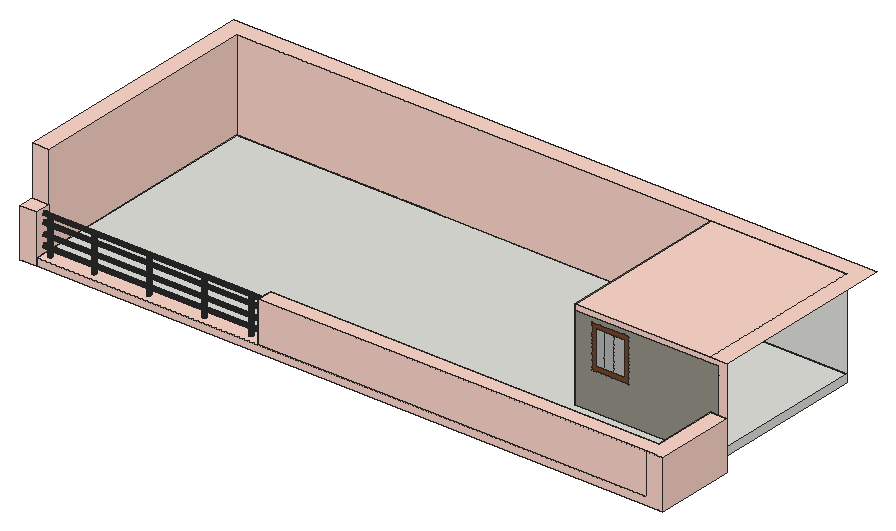
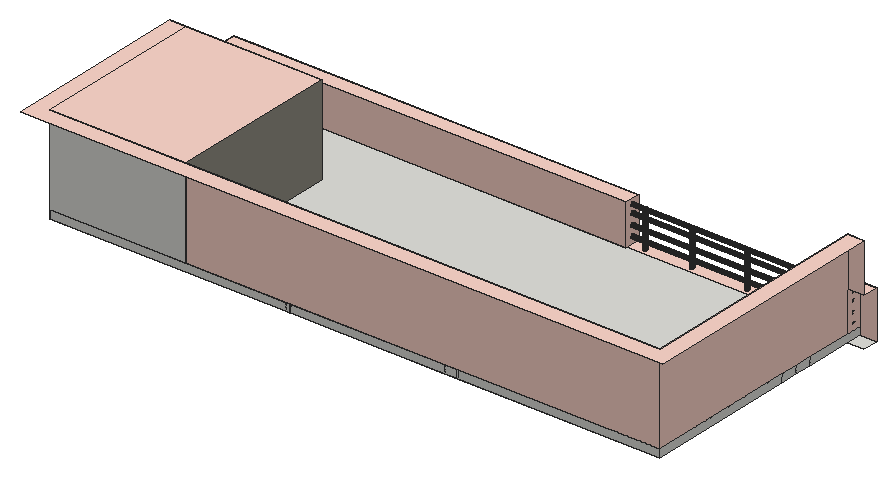
# SketchUp Ruby script. Lengths in inches.
U = 1.inch
M = Sketchup.active_model
def pt(a) = Geom::Point3d.new(a.map { |v| v * U })
def face(e, loops, mat)
  f = e.add_face(loops[0].map { |a| pt(a) })
  loops[1..].each { |l| e.add_face(l.map { |a| pt(a) }).erase! }
  f.material = f.back_material = mat if mat
  f
end
# faces: each face lists its corners as indices into pts; further lists are holes
def faces(e, pts, list, mat = nil) = list.each { |f| face(e, (f[0].is_a?(Array) ? f : [f]).map { |l| l.map { |i| pts[i] } }, mat) }
# xy, xz, yz: faces in a plane at the given z, y or x. An outline is a flat list of corners, or four numbers for a rectangle; further outlines are holes
def ring(l) = l.size == 4 ? [[l[0], l[1]], [l[2], l[1]], [l[2], l[3]], [l[0], l[3]]] : l.each_slice(2).to_a
def flat(e, list, mat, &to3) = list.each { |f| face(e, (f[0].is_a?(Array) ? f : [f]).map { |l| ring(l).map { |u, v| to3.(u, v) } }, mat) }
def xy(e, z, list, mat = nil) = flat(e, list, mat) { |x, y| [x, y, z] }
def xz(e, y, list, mat = nil) = flat(e, list, mat) { |x, z| [x, y, z] }
def yz(e, x, list, mat = nil) = flat(e, list, mat) { |y, z| [x, y, z] }
def lines(e, pts, list) = list.each { |a, b| e.add_line(pt(pts[a]), pt(pts[b])) }
# prism: a flat outline (further loops are holes) pulled along v
def prism(e, loops, v, mat = nil)
  f = face(e, loops, mat); d = Geom::Vector3d.new(v.map { |x| x * U })
  f.pushpull(f.normal.samedirection?(d) ? d.length : -d.length)
end
def box(e, o, s, mat = nil) = prism(e, [[o, [o[0] + s[0], o[1], o[2]], [o[0] + s[0], o[1] + s[1], o[2]], [o[0], o[1] + s[1], o[2]]]], [0, 0, s[2]], mat)
def at(x, y, z, deg = 0) = Geom::Transformation.translation(pt([x, y, z])) * Geom::Transformation.rotation(ORIGIN, Z_AXIS, deg.degrees)
def axes(o, x, y, z) = Geom::Transformation.new([*x, 0, *y, 0, *z, 0, *pt(o).to_a, 1])
def part(name) = M.definitions.add(name)
# library, detail: a bought-in or finely detailed component or shape, given as its bounding box
def library(name, o, s) = part(name).tap { |d| box(d.entities, o, s) }
def detail(e, o, s) = box(e.add_group.entities, o, s)
def put(e, d, t, mat = nil) = e.add_instance(d, t).tap { |i| i.material = mat if mat }
def group(e, t, mat = nil) = e.add_group.tap { |g| g.transformation = t; g.material = mat if mat }.entities
root = M.entities
M.materials.add("[Color B01]").color = [255, 216, 204]
M.materials.add("[Formica Graystone]").color = [149, 146, 135]
M.materials.add("[Formica Laminate Dark]").color = [50, 53, 60]
M.materials.add("[Mirror 01]").color = [185, 185, 185]
M.materials.add("[Wood Veneer 01]1").color = [120, 70, 37]
xy(root,2577.9375,[[0,195.0625,77.93,267.5625],[77.93,571.9,1096.47,653.97],[1096.47,571.9,1845.89,653.97],[1845.89,571.9,2962.22,653.97],[77.93,653.97,1096.47,1377.24],
  [1096.47,653.97,1845.89,1377.24],[1845.89,653.97,2962.22,1377.24]])
xy(root,2577.9375,[[[77.93,195.0625,2962.22,571.9],[95.12,236.1875,148.18,267.5625],[180.68,236.1875,233.75,267.5625],[265.56,236.1875,318.62,267.5625],[352.87,236.1875,405.93,267.5625]],[2962.22,195.0625,3040.15,571.9]],"[Color B01]")
xy(root,2613.9375,[[1125.51,195.0625,2962.22,267.5625],[112.1,225.43,109.76,225.74,107.57,226.65,105.7,228.09,104.25,229.96,103.35,232.15,103.04,234.5,103.35,236.84,104.25,239.03,105.7,240.9,107.57,242.34,109.76,243.25,112.1,243.56,114.45,243.25,116.63,242.34,118.51,240.9,119.95,239.03,120.86,236.84,121.17,234.5,120.86,232.15,119.95,229.96,118.51,228.09,116.63,226.65,114.45,225.74],[318.54,225.43,316.2,225.74,314.01,226.65,312.13,228.09,310.69,229.96,309.79,232.15,309.48,234.5,309.79,236.84,310.69,239.03,312.13,240.9,314.01,242.34,316.2,243.25,318.54,243.56,320.89,243.25,323.07,242.34,324.95,240.9,326.39,239.03,327.29,236.84,327.6,234.5,327.29,232.15,326.39,229.96,324.95,228.09,323.07,226.65,320.89,225.74],[577.42,225.43,575.07,225.74,572.88,226.65,571.01,228.09,569.57,229.96,568.66,232.15,568.35,234.5,568.66,236.84,569.57,239.03,571.01,240.9,572.88,242.34,575.07,243.25,577.42,243.56,579.76,243.25,581.95,242.34,583.82,240.9,585.26,239.03,586.17,236.84,586.48,234.5,586.17,232.15,585.26,229.96,583.82,228.09,581.95,226.65,579.76,225.74],[840.42,225.43,838.07,225.74,835.88,226.65,834.01,228.09,832.57,229.96,831.66,232.15,831.35,234.5,831.66,236.84,832.57,239.03,834.01,240.9,835.88,242.34,838.07,243.25,840.42,243.56,842.76,243.25,844.95,242.34,846.82,240.9,848.26,239.03,849.17,236.84,849.48,234.5,849.17,232.15,848.26,229.96,846.82,228.09,844.95,226.65,842.76,225.74],
  [1060.29,225.43,1057.95,225.74,1055.76,226.65,1053.88,228.09,1052.44,229.96,1051.54,232.15,1051.23,234.5,1051.54,236.84,1052.44,239.03,1053.88,240.9,1055.76,242.34,1057.95,243.25,1060.29,243.56,1062.64,243.25,1064.82,242.34,1066.7,240.9,1068.14,239.03,1069.04,236.84,1069.35,234.5,1069.04,232.15,1068.14,229.96,1066.7,228.09,1064.82,226.65,1062.64,225.74],[77.93,267.5625,2962.22,267.5625,2962.22,571.9,2321.78,571.9,2321.78,1377.24,77.93,1377.24],[2321.78,571.9,2962.22,653.97],[2321.78,653.97,2962.22,1377.24]])
xy(root,2613.9375,[[[77.93,195.0625,1125.51,267.5625],[112.1,225.43,109.76,225.74,107.57,226.65,105.7,228.09,104.25,229.96,103.35,232.15,103.04,234.5,103.35,236.84,104.25,239.03,105.7,240.9,107.57,242.34,109.76,243.25,112.1,243.56,114.45,243.25,116.63,242.34,118.51,240.9,119.95,239.03,120.86,236.84,121.17,234.5,120.86,232.15,119.95,229.96,118.51,228.09,116.63,226.65,114.45,225.74],[1060.29,225.43,1057.95,225.74,1055.76,226.65,1053.88,228.09,1052.44,229.96,1051.54,232.15,1051.23,234.5,1051.54,236.84,1052.44,239.03,1053.88,240.9,1055.76,242.34,1057.95,243.25,1060.29,243.56,1062.64,243.25,1064.82,242.34,1066.7,240.9,1068.14,239.03,1069.04,236.84,1069.35,234.5,1069.04,232.15,1068.14,229.96,1066.7,228.09,1064.82,226.65,1062.64,225.74],[318.54,225.43,316.2,225.74,314.01,226.65,312.13,228.09,310.69,229.96,309.79,232.15,309.48,234.5,309.79,236.84,310.69,239.03,312.13,240.9,314.01,242.34,316.2,243.25,318.54,243.56,320.89,243.25,323.07,242.34,324.95,240.9,326.39,239.03,327.29,236.84,327.6,234.5,327.29,232.15,326.39,229.96,324.95,228.09,323.07,226.65,320.89,225.74],[840.42,225.43,838.07,225.74,835.88,226.65,834.01,228.09,832.57,229.96,831.66,232.15,831.35,234.5,831.66,236.84,832.57,239.03,834.01,240.9,835.88,242.34,838.07,243.25,840.42,243.56,842.76,243.25,844.95,242.34,846.82,240.9,848.26,239.03,849.17,236.84,849.48,234.5,849.17,232.15,848.26,229.96,846.82,228.09,844.95,226.65,842.76,225.74],[577.42,225.43,575.07,225.74,572.88,226.65,571.01,228.09,569.57,229.96,568.66,232.15,568.35,234.5,568.66,236.84,569.57,239.03,571.01,240.9,572.88,242.34,575.07,243.25,577.42,243.56,579.76,243.25,581.95,242.34,583.82,240.9,585.26,239.03,586.17,236.84,586.48,234.5,586.17,232.15,585.26,229.96,583.82,228.09,581.95,226.65,579.76,225.74]]],"[Color B01]")
xy(root,2782.1875,[[840.42,225.43,842.76,225.74,844.95,226.65,846.82,228.09,848.26,229.96,849.17,232.15,849.48,234.5,849.17,236.84,848.26,239.03,846.82,240.9,844.95,242.34,842.76,243.25,840.42,243.56,838.07,243.25,835.88,242.34,834.01,240.9,832.57,239.03,831.66,236.84,831.35,234.5,831.66,232.15,832.57,229.96,834.01,228.09,835.88,226.65,838.07,225.74]])
xy(root,2783.625,[[577.42,225.43,579.76,225.74,581.95,226.65,583.82,228.09,585.26,229.96,586.17,232.15,586.48,234.5,586.17,236.84,585.26,239.03,583.82,240.9,581.95,242.34,579.76,243.25,577.42,243.56,575.07,243.25,572.88,242.34,571.01,240.9,569.57,239.03,568.66,236.84,568.35,234.5,568.66,232.15,569.57,229.96,571.01,228.09,572.88,226.65,575.07,225.74]])
xy(root,2783.6875,[[318.54,225.43,320.89,225.74,323.07,226.65,324.95,228.09,326.39,229.96,327.29,232.15,327.6,234.5,327.29,236.84,326.39,239.03,324.95,240.9,323.07,242.34,320.89,243.25,318.54,243.56,316.2,243.25,314.01,242.34,312.13,240.9,310.69,239.03,309.79,236.84,309.48,234.5,309.79,232.15,310.69,229.96,312.13,228.09,314.01,226.65,316.2,225.74]])
xy(root,2783.875,[[112.1,225.43,114.45,225.74,116.63,226.65,118.51,228.09,119.95,229.96,120.86,232.15,121.17,234.5,120.86,236.84,119.95,239.03,118.51,240.9,116.63,242.34,114.45,243.25,112.1,243.56,109.76,243.25,107.57,242.34,105.7,240.9,104.25,239.03,103.35,236.84,103.04,234.5,103.35,232.15,104.25,229.96,105.7,228.09,107.57,226.65,109.76,225.74]])
xy(root,2789.06,[[1060.29,225.43,1062.64,225.74,1064.82,226.65,1066.58,227.99,1054.01,227.99,1055.76,226.65,1057.95,225.74],[1054.01,227.99,1066.58,227.99,1066.7,228.09,1068.14,229.96,1069.04,232.15,1069.35,234.5,1069.04,236.84,1068.14,239.03,1066.7,240.9,1065.04,242.17,1055.54,242.17,1053.88,240.9,1052.44,239.03,1051.54,236.84,1051.23,234.5,1051.54,232.15,1052.44,229.96,1053.88,228.09],[1055.54,242.17,1065.04,242.17,1064.82,242.34,1062.64,243.25,1060.29,243.56,1057.95,243.25,1055.76,242.34]])
xy(root,2806.5,[[0,195.0625,77.93,267.5625],[1125.51,195.0625,3040.15,195.0625,3040.15,571.9,2962.22,571.9,2962.22,267.5625,1125.51,267.5625]],"[Color B01]")
xy(root,3039.125,[[0,267.5625,77.93,267.5625,77.93,1377.24,2962.22,1377.24,2962.22,571.9,3040.15,571.9,3040.15,1455.17,0,1455.17],[2321.78,571.9,2962.22,1377.24]],"[Color B01]")
xz(root,195.0625,[[0,2577.9375,77.93,2806.5],[77.93,2577.9375,3040.15,2577.9375,3040.15,2806.5,2962.22,2806.5,2962.22,2613.9375,77.93,2613.9375],[1125.51,2613.9375,2962.22,2806.5]],"[Color B01]")
xz(root,267.5625,[[1125.51,2613.9375,2962.22,2806.5],[0,2806.5,77.93,3039.125]],"[Color B01]")
xz(root,571.9,[[2962.22,2577.9375,3040.15,2806.5]])
xz(root,571.9,[[3000.97,2806.5,3040.15,2806.5,3040.15,3039.125,2321.78,3039.125,2321.78,3014.36,3000.97,3014.36]],"[Color B01]")
xz(root,571.9,[[[2321.78,2613.9375,2962.22,2613.9375,2962.22,2806.5,3000.97,2806.5,3000.97,3014.36,2321.78,3014.36],[2400.23,2788.12,2578.04,2993.56]]],"[Formica Graystone]")
xz(root,571.9,[[2424.88,2812.78,2458.58,2968.9],[2458.58,2812.78,2505.98,2968.9],[2505.98,2812.78,2553.38,2968.9]],"[Mirror 01]")
xz(root,571.9,[[[2400.23,2788.12,2578.04,2993.56],[2424.88,2812.78,2553.38,2968.9]]],"[Wood Veneer 01]1")
xz(root,1377.24,[[77.93,2577.9375,1031.89,2613.9375],[1031.89,2577.9375,1038.88,2613.9375],[1038.88,2577.9375,1096.47,2613.9375],[1096.47,2577.9375,1822.57,2613.9375],[1822.57,2577.9375,1828.6875,2613.9375],
  [1828.6875,2577.9375,1845.89,2613.9375],[1845.89,2577.9375,2962.22,2613.9375],[2321.78,2613.9375,2962.22,3039.125]])
xz(root,1377.24,[[77.93,2613.9375,2321.78,3039.125]],"[Color B01]")
yz(root,77.93,[[195.0625,2577.9375,488.625,2613.9375],[488.625,2577.9375,571.9,2613.9375],[571.9,2577.9375,653.97,2613.9375],[653.97,2577.9375,1377.24,2613.9375]])
yz(root,77.93,[[[195.0625,2613.9375,267.5625,2806.5],[235.08,2776.78,232.96,2777.06,230.99,2777.875,229.29,2779.18,227.99,2780.87,227.17,2782.85,226.9,2784.97,227.17,2787.08,227.99,2789.06,229.29,2790.75,230.99,2792.06,232.96,2792.875,235.08,2793.15,237.2,2792.875,239.18,2792.06,240.87,2790.75,242.17,2789.06,242.99,2787.08,243.27,2784.97,242.99,2782.85,242.17,2780.87,240.87,2779.18,239.18,2777.875,237.2,2777.06],[235.08,2738.47,232.96,2738.74,230.99,2739.5625,229.29,2740.86,227.99,2742.56,227.17,2744.53,226.9,2746.65,227.17,2748.77,227.99,2750.75,229.29,2752.44,230.99,2753.74,232.96,2754.5625,235.08,2754.84,237.2,2754.5625,239.18,2753.74,240.87,2752.44,242.17,2750.75,242.99,2748.77,243.27,2746.65,242.99,2744.53,242.17,2742.56,240.87,2740.86,239.18,2739.5625,237.2,2738.74],[235.08,2688.47,232.96,2688.74,230.99,2689.5625,229.29,2690.86,227.99,2692.56,227.17,2694.53,226.9,2696.65,227.17,2698.77,227.99,2700.75,229.29,2702.44,230.99,2703.74,232.96,2704.5625,235.08,2704.84,237.2,2704.5625,239.18,2703.74,240.87,2702.44,242.17,2700.75,242.99,2698.77,243.27,2696.65,242.99,2694.53,242.17,2692.56,240.87,2690.86,239.18,2689.5625,237.2,2688.74],[235.08,2639.53,232.96,2639.81,230.99,2640.625,229.29,2641.93,227.99,2643.62,227.17,2645.6,226.9,2647.72,227.17,2649.83,227.99,2651.81,229.29,2653.5,230.99,2654.81,232.96,2655.625,235.08,2655.9,237.2,2655.625,239.18,2654.81,240.87,2653.5,242.17,2651.81,242.99,2649.83,243.27,2647.72,242.99,2645.6,242.17,2643.62,240.87,2641.93,239.18,2640.625,237.2,2639.81]],[267.5625,2613.9375,1377.24,3039.125]],"[Color B01]")
yz(root,1125.51,[[235.08,2639.53,237.2,2639.81,239.18,2640.625,240.87,2641.93,242.17,2643.62,242.99,2645.6,243.27,2647.72,242.99,2649.83,242.17,2651.81,240.87,2653.5,239.18,2654.81,237.2,2655.625,235.08,2655.9,232.96,2655.625,230.99,2654.81,229.29,2653.5,227.99,2651.81,227.17,2649.83,226.9,2647.72,227.17,2645.6,227.99,2643.62,229.29,2641.93,230.99,2640.625,232.96,2639.81],[235.08,2688.47,237.2,2688.74,239.18,2689.5625,240.87,2690.86,242.17,2692.56,242.99,2694.53,243.27,2696.65,242.99,2698.77,242.17,2700.75,240.87,2702.44,239.18,2703.74,237.2,2704.5625,235.08,2704.84,232.96,2704.5625,230.99,2703.74,229.29,2702.44,227.99,2700.75,227.17,2698.77,226.9,2696.65,227.17,2694.53,227.99,2692.56,229.29,2690.86,230.99,2689.5625,232.96,2688.74],[235.08,2738.47,237.2,2738.74,239.18,2739.5625,240.87,2740.86,242.17,2742.56,242.99,2744.53,243.27,2746.65,242.99,2748.77,242.17,2750.75,240.87,2752.44,239.18,2753.74,237.2,2754.5625,235.08,2754.84,232.96,2754.5625,230.99,2753.74,229.29,2752.44,227.99,2750.75,227.17,2748.77,226.9,2746.65,227.17,2744.53,227.99,2742.56,229.29,2740.86,230.99,2739.5625,232.96,2738.74],[235.08,2776.78,237.2,2777.06,239.18,2777.875,240.87,2779.18,242.17,2780.87,242.99,2782.85,243.27,2784.97,242.99,2787.08,242.17,2789.06,240.87,2790.75,239.18,2792.06,237.2,2792.875,235.08,2793.15,232.96,2792.875,230.99,2792.06,229.29,2790.75,227.99,2789.06,227.17,2787.08,226.9,2784.97,227.17,2782.85,227.99,2780.87,229.29,2779.18,230.99,2777.875,232.96,2777.06]])
yz(root,1125.51,[[[195.0625,2613.9375,267.5625,2806.5],[235.08,2776.78,237.2,2777.06,239.18,2777.875,240.87,2779.18,242.17,2780.87,242.99,2782.85,243.27,2784.97,242.99,2787.08,242.17,2789.06,240.87,2790.75,239.18,2792.06,237.2,2792.875,235.08,2793.15,232.96,2792.875,230.99,2792.06,229.29,2790.75,227.99,2789.06,227.17,2787.08,226.9,2784.97,227.17,2782.85,227.99,2780.87,229.29,2779.18,230.99,2777.875,232.96,2777.06],[235.08,2639.53,237.2,2639.81,239.18,2640.625,240.87,2641.93,242.17,2643.62,242.99,2645.6,243.27,2647.72,242.99,2649.83,242.17,2651.81,240.87,2653.5,239.18,2654.81,237.2,2655.625,235.08,2655.9,232.96,2655.625,230.99,2654.81,229.29,2653.5,227.99,2651.81,227.17,2649.83,226.9,2647.72,227.17,2645.6,227.99,2643.62,229.29,2641.93,230.99,2640.625,232.96,2639.81],[235.08,2738.47,237.2,2738.74,239.18,2739.5625,240.87,2740.86,242.17,2742.56,242.99,2744.53,243.27,2746.65,242.99,2748.77,242.17,2750.75,240.87,2752.44,239.18,2753.74,237.2,2754.5625,235.08,2754.84,232.96,2754.5625,230.99,2753.74,229.29,2752.44,227.99,2750.75,227.17,2748.77,226.9,2746.65,227.17,2744.53,227.99,2742.56,229.29,2740.86,230.99,2739.5625,232.96,2738.74],[235.08,2688.47,237.2,2688.74,239.18,2689.5625,240.87,2690.86,242.17,2692.56,242.99,2694.53,243.27,2696.65,242.99,2698.77,242.17,2700.75,240.87,2702.44,239.18,2703.74,237.2,2704.5625,235.08,2704.84,232.96,2704.5625,230.99,2703.74,229.29,2702.44,227.99,2700.75,227.17,2698.77,226.9,2696.65,227.17,2694.53,227.99,2692.56,229.29,2690.86,230.99,2689.5625,232.96,2688.74]]],"[Color B01]")
yz(root,2321.78,[[571.9,2613.9375,1377.24,3039.125]],"[Formica Graystone]")
yz(root,2962.22,[[571.9,2577.9375,653.97,2613.9375],[653.97,2577.9375,1377.24,2613.9375]])
yz(root,2962.22,[[267.5625,2613.9375,571.9,2806.5]],"[Color B01]")
yz(root,3040.15,[[195.0625,2577.9375,571.9,2806.5]],"[Color B01]")
p = [[109.76,225.74,2613.9375],[112.1,225.43,2613.9375],[112.1,225.43,2783.875],[109.76,225.74,2783.875],[114.45,225.74,2613.9375],[114.45,225.74,2783.875],
  [316.2,225.74,2613.9375],[318.54,225.43,2613.9375],[318.54,225.43,2783.6875],[316.2,225.74,2783.6875],[320.89,225.74,2613.9375],[320.89,225.74,2783.6875],
  [575.07,225.74,2613.9375],[577.42,225.43,2613.9375],[577.42,225.43,2783.625],[575.07,225.74,2783.625],[579.76,225.74,2613.9375],[579.76,225.74,2783.625],
  [838.07,225.74,2613.9375],[840.42,225.43,2613.9375],[840.42,225.43,2782.1875],[838.07,225.74,2782.1875],[842.76,225.74,2613.9375],[842.76,225.74,2782.1875],
  [1057.95,225.74,2613.9375],[1060.29,225.43,2613.9375],[1060.29,225.43,2789.06],[1057.95,225.74,2789.06],[1062.64,225.74,2613.9375],[1062.64,225.74,2789.06],
  [107.57,226.65,2613.9375],[107.57,226.65,2783.875],[116.63,226.65,2613.9375],[116.63,226.65,2783.875],[314.01,226.65,2613.9375],[314.01,226.65,2783.6875],
  [323.07,226.65,2613.9375],[323.07,226.65,2783.6875],[572.88,226.65,2613.9375],[572.88,226.65,2783.625],[581.95,226.65,2613.9375],[581.95,226.65,2783.625],
  [835.88,226.65,2613.9375],[835.88,226.65,2782.1875],[844.95,226.65,2613.9375],[844.95,226.65,2782.1875],[1055.76,226.65,2613.9375],[1055.76,226.65,2789.06],
  [1064.82,226.65,2613.9375],[1064.82,226.65,2789.06],[105.7,228.09,2613.9375],[105.7,228.09,2783.875],[118.51,228.09,2613.9375],[118.51,228.09,2783.875],
  [312.13,228.09,2613.9375],[312.13,228.09,2783.6875],[324.95,228.09,2613.9375],[324.95,228.09,2783.6875],[571.01,228.09,2613.9375],[571.01,228.09,2783.625],
  [583.82,228.09,2613.9375],[583.82,228.09,2783.625],[834.01,228.09,2613.9375],[834.01,228.09,2782.1875],[846.82,228.09,2613.9375],[846.82,228.09,2782.1875],
  [1053.88,228.09,2613.9375],[1054.01,227.99,2789.06],[1053.88,228.09,2789.06],[1066.7,228.09,2613.9375],[1066.7,228.09,2789.06],[1066.58,227.99,2789.06],
  [104.25,229.96,2613.9375],[104.25,229.96,2783.875],[119.95,229.96,2613.9375],[119.95,229.96,2783.875],[310.69,229.96,2613.9375],[310.69,229.96,2783.6875],
  [326.39,229.96,2613.9375],[326.39,229.96,2783.6875],[569.57,229.96,2613.9375],[569.57,229.96,2783.625],[585.26,229.96,2613.9375],[585.26,229.96,2783.625],
  [832.57,229.96,2613.9375],[832.57,229.96,2782.1875],[848.26,229.96,2613.9375],[848.26,229.96,2782.1875],[1052.44,229.96,2613.9375],[1052.44,229.96,2789.06],
  [1068.14,229.96,2613.9375],[1068.14,229.96,2789.06],[103.35,232.15,2613.9375],[103.35,232.15,2783.875],[120.86,232.15,2613.9375],[120.86,232.15,2783.875],
  [309.79,232.15,2613.9375],[309.79,232.15,2783.6875],[327.29,232.15,2613.9375],[327.29,232.15,2783.6875],[568.66,232.15,2613.9375],[568.66,232.15,2783.625],
  [586.17,232.15,2613.9375],[586.17,232.15,2783.625],[831.66,232.15,2613.9375],[831.66,232.15,2782.1875],[849.17,232.15,2613.9375],[849.17,232.15,2782.1875],
  [1051.54,232.15,2613.9375],[1051.54,232.15,2789.06],[1069.04,232.15,2613.9375],[1069.04,232.15,2789.06],[103.04,234.5,2613.9375],[103.04,234.5,2783.875],
  [121.17,234.5,2613.9375],[121.17,234.5,2783.875],[309.48,234.5,2613.9375],[309.48,234.5,2783.6875],[327.6,234.5,2613.9375],[327.6,234.5,2783.6875],
  [568.35,234.5,2613.9375],[568.35,234.5,2783.625],[586.48,234.5,2613.9375],[586.48,234.5,2783.625],[831.35,234.5,2613.9375],[831.35,234.5,2782.1875],
  [849.48,234.5,2613.9375],[849.48,234.5,2782.1875],[1051.23,234.5,2613.9375],[1051.23,234.5,2789.06],[1069.35,234.5,2613.9375],[1069.35,234.5,2789.06],
  [103.35,236.84,2613.9375],[103.35,236.84,2783.875],[120.86,236.84,2613.9375],[120.86,236.84,2783.875],[309.79,236.84,2613.9375],[309.79,236.84,2783.6875],
  [327.29,236.84,2613.9375],[327.29,236.84,2783.6875],[568.66,236.84,2613.9375],[568.66,236.84,2783.625],[586.17,236.84,2613.9375],[586.17,236.84,2783.625],
  [831.66,236.84,2613.9375],[831.66,236.84,2782.1875],[849.17,236.84,2613.9375],[849.17,236.84,2782.1875],[1051.54,236.84,2613.9375],[1051.54,236.84,2789.06],
  [1069.04,236.84,2613.9375],[1069.04,236.84,2789.06],[104.25,239.03,2613.9375],[104.25,239.03,2783.875],[119.95,239.03,2613.9375],[119.95,239.03,2783.875],
  [310.69,239.03,2613.9375],[310.69,239.03,2783.6875],[326.39,239.03,2613.9375],[326.39,239.03,2783.6875],[569.57,239.03,2613.9375],[569.57,239.03,2783.625],
  [585.26,239.03,2613.9375],[585.26,239.03,2783.625],[832.57,239.03,2613.9375],[832.57,239.03,2782.1875],[848.26,239.03,2613.9375],[848.26,239.03,2782.1875],
  [1052.44,239.03,2613.9375],[1052.44,239.03,2789.06],[1068.14,239.03,2613.9375],[1068.14,239.03,2789.06],[105.7,240.9,2613.9375],[105.7,240.9,2783.875],
  [118.51,240.9,2613.9375],[118.51,240.9,2783.875],[312.13,240.9,2613.9375],[312.13,240.9,2783.6875],[324.95,240.9,2613.9375],[324.95,240.9,2783.6875],
  [571.01,240.9,2613.9375],[571.01,240.9,2783.625],[583.82,240.9,2613.9375],[583.82,240.9,2783.625],[834.01,240.9,2613.9375],[834.01,240.9,2782.1875],
  [846.82,240.9,2613.9375],[846.82,240.9,2782.1875],[1053.88,240.9,2613.9375],[1053.88,240.9,2789.06],[1066.7,240.9,2613.9375],[1066.7,240.9,2789.06],
  [107.57,242.34,2613.9375],[107.57,242.34,2783.875],[116.63,242.34,2613.9375],[116.63,242.34,2783.875],[314.01,242.34,2613.9375],[314.01,242.34,2783.6875],
  [323.07,242.34,2613.9375],[323.07,242.34,2783.6875],[572.88,242.34,2613.9375],[572.88,242.34,2783.625],[581.95,242.34,2613.9375],[581.95,242.34,2783.625],
  [835.88,242.34,2613.9375],[835.88,242.34,2782.1875],[844.95,242.34,2613.9375],[844.95,242.34,2782.1875],[1055.76,242.34,2613.9375],[1055.54,242.17,2789.06],
  [1055.76,242.34,2789.06],[1064.82,242.34,2613.9375],[1064.82,242.34,2789.06],[1065.04,242.17,2789.06],[109.76,243.25,2613.9375],[109.76,243.25,2783.875],
  [114.45,243.25,2613.9375],[114.45,243.25,2783.875],[316.2,243.25,2613.9375],[316.2,243.25,2783.6875],[320.89,243.25,2613.9375],[320.89,243.25,2783.6875],
  [575.07,243.25,2613.9375],[575.07,243.25,2783.625],[579.76,243.25,2613.9375],[579.76,243.25,2783.625],[838.07,243.25,2613.9375],[838.07,243.25,2782.1875],
  [842.76,243.25,2613.9375],[842.76,243.25,2782.1875],[1057.95,243.25,2613.9375],[1057.95,243.25,2789.06],[1062.64,243.25,2613.9375],[1062.64,243.25,2789.06],
  [112.1,243.56,2613.9375],[112.1,243.56,2783.875],[318.54,243.56,2613.9375],[318.54,243.56,2783.6875],[577.42,243.56,2613.9375],[577.42,243.56,2783.625],
  [840.42,243.56,2613.9375],[840.42,243.56,2782.1875],[1060.29,243.56,2613.9375],[1060.29,243.56,2789.06],[1125.51,235.08,2639.53],[1125.51,232.96,2639.81],
  [77.93,232.96,2639.81],[77.93,235.08,2639.53],[1125.51,237.2,2639.81],[77.93,237.2,2639.81],[1125.51,230.99,2640.625],[77.93,230.99,2640.625],
  [1125.51,239.18,2640.625],[77.93,239.18,2640.625],[1125.51,229.29,2641.93],[77.93,229.29,2641.93],[1125.51,240.87,2641.93],[77.93,240.87,2641.93],
  [1125.51,227.99,2643.62],[77.93,227.99,2643.62],[1125.51,242.17,2643.62],[77.93,242.17,2643.62],[1125.51,227.17,2645.6],[77.93,227.17,2645.6],
  [1125.51,242.99,2645.6],[77.93,242.99,2645.6],[1125.51,226.9,2647.72],[77.93,226.9,2647.72],[1125.51,243.27,2647.72],[77.93,243.27,2647.72],
  [1125.51,227.17,2649.83],[77.93,227.17,2649.83],[1125.51,242.99,2649.83],[77.93,242.99,2649.83],[1125.51,227.99,2651.81],[77.93,227.99,2651.81],
  [1125.51,242.17,2651.81],[77.93,242.17,2651.81],[1125.51,229.29,2653.5],[77.93,229.29,2653.5],[1125.51,240.87,2653.5],[77.93,240.87,2653.5],
  [1125.51,230.99,2654.81],[77.93,230.99,2654.81],[1125.51,239.18,2654.81],[77.93,239.18,2654.81],[1125.51,232.96,2655.625],[77.93,232.96,2655.625],
  [1125.51,237.2,2655.625],[77.93,237.2,2655.625],[1125.51,235.08,2655.9],[77.93,235.08,2655.9],[1125.51,235.08,2688.47],[1125.51,232.96,2688.74],
  [77.93,232.96,2688.74],[77.93,235.08,2688.47],[1125.51,237.2,2688.74],[77.93,237.2,2688.74],[1125.51,230.99,2689.5625],[77.93,230.99,2689.5625],
  [1125.51,239.18,2689.5625],[77.93,239.18,2689.5625],[1125.51,229.29,2690.86],[77.93,229.29,2690.86],[1125.51,240.87,2690.86],[77.93,240.87,2690.86],
  [1125.51,227.99,2692.56],[77.93,227.99,2692.56],[1125.51,242.17,2692.56],[77.93,242.17,2692.56],[1125.51,227.17,2694.53],[77.93,227.17,2694.53],
  [1125.51,242.99,2694.53],[77.93,242.99,2694.53],[1125.51,226.9,2696.65],[77.93,226.9,2696.65],[1125.51,243.27,2696.65],[77.93,243.27,2696.65],
  [1125.51,227.17,2698.77],[77.93,227.17,2698.77],[1125.51,242.99,2698.77],[77.93,242.99,2698.77],[1125.51,227.99,2700.75],[77.93,227.99,2700.75],
  [1125.51,242.17,2700.75],[77.93,242.17,2700.75],[1125.51,229.29,2702.44],[77.93,229.29,2702.44],[1125.51,240.87,2702.44],[77.93,240.87,2702.44],
  [1125.51,230.99,2703.74],[77.93,230.99,2703.74],[1125.51,239.18,2703.74],[77.93,239.18,2703.74],[1125.51,232.96,2704.5625],[77.93,232.96,2704.5625],
  [1125.51,237.2,2704.5625],[77.93,237.2,2704.5625],[1125.51,235.08,2704.84],[77.93,235.08,2704.84],[1125.51,235.08,2738.47],[1125.51,232.96,2738.74],
  [77.93,232.96,2738.74],[77.93,235.08,2738.47],[1125.51,237.2,2738.74],[77.93,237.2,2738.74],[1125.51,230.99,2739.5625],[77.93,230.99,2739.5625],
  [1125.51,239.18,2739.5625],[77.93,239.18,2739.5625],[1125.51,229.29,2740.86],[77.93,229.29,2740.86],[1125.51,240.87,2740.86],[77.93,240.87,2740.86],
  [1125.51,227.99,2742.56],[77.93,227.99,2742.56],[1125.51,242.17,2742.56],[77.93,242.17,2742.56],[1125.51,227.17,2744.53],[77.93,227.17,2744.53],
  [1125.51,242.99,2744.53],[77.93,242.99,2744.53],[1125.51,226.9,2746.65],[77.93,226.9,2746.65],[1125.51,243.27,2746.65],[77.93,243.27,2746.65],
  [1125.51,227.17,2748.77],[77.93,227.17,2748.77],[1125.51,242.99,2748.77],[77.93,242.99,2748.77],[1125.51,227.99,2750.75],[77.93,227.99,2750.75],
  [1125.51,242.17,2750.75],[77.93,242.17,2750.75],[1125.51,229.29,2752.44],[77.93,229.29,2752.44],[1125.51,240.87,2752.44],[77.93,240.87,2752.44],
  [1125.51,230.99,2753.74],[77.93,230.99,2753.74],[1125.51,239.18,2753.74],[77.93,239.18,2753.74],[1125.51,232.96,2754.5625],[77.93,232.96,2754.5625],
  [1125.51,237.2,2754.5625],[77.93,237.2,2754.5625],[1125.51,235.08,2754.84],[77.93,235.08,2754.84],[1125.51,235.08,2776.78],[1125.51,232.96,2777.06],
  [77.93,232.96,2777.06],[77.93,235.08,2776.78],[1125.51,237.2,2777.06],[77.93,237.2,2777.06],[1125.51,230.99,2777.875],[77.93,230.99,2777.875],
  [1125.51,239.18,2777.875],[77.93,239.18,2777.875],[1125.51,229.29,2779.18],[77.93,229.29,2779.18],[1125.51,240.87,2779.18],[77.93,240.87,2779.18],
  [1125.51,227.99,2780.87],[77.93,227.99,2780.87],[1125.51,242.17,2780.87],[77.93,242.17,2780.87],[1125.51,227.17,2782.85],[77.93,227.17,2782.85],
  [1125.51,242.99,2782.85],[77.93,242.99,2782.85],[1125.51,226.9,2784.97],[77.93,226.9,2784.97],[1125.51,243.27,2784.97],[77.93,243.27,2784.97],
  [1125.51,227.17,2787.08],[77.93,227.17,2787.08],[1125.51,242.99,2787.08],[77.93,242.99,2787.08],[1125.51,227.99,2789.06],[77.93,227.99,2789.06],
  [1125.51,242.17,2789.06],[77.93,242.17,2789.06],[1125.51,229.29,2790.75],[77.93,229.29,2790.75],[1125.51,240.87,2790.75],[77.93,240.87,2790.75],
  [1125.51,230.99,2792.06],[77.93,230.99,2792.06],[1125.51,239.18,2792.06],[77.93,239.18,2792.06],[1125.51,232.96,2792.875],[77.93,232.96,2792.875],
  [1125.51,237.2,2792.875],[77.93,237.2,2792.875],[1125.51,235.08,2793.15],[77.93,235.08,2793.15]]
faces(root,p,[[0,1,2,3],[1,4,5,2],[6,7,8,9],[7,10,11,8],[12,13,14,15],[13,16,17,14],[18,19,20,21],[19,22,23,20],
  [24,25,26,27],[25,28,29,26],[30,0,3,31],[4,32,33,5],[34,6,9,35],[10,36,37,11],[38,12,15,39],[16,40,41,17],
  [42,18,21,43],[22,44,45,23],[46,24,27,47],[28,48,49,29],[50,30,31,51],[32,52,53,33],[54,34,35,55],[36,56,57,37],
  [58,38,39,59],[40,60,61,41],[62,42,43,63],[44,64,65,45],[66,46,47,67,68],[48,69,70,71,49],[72,50,51,73],[52,74,75,53],
  [76,54,55,77],[56,78,79,57],[80,58,59,81],[60,82,83,61],[84,62,63,85],[64,86,87,65],[88,66,68,89],[69,90,91,70],
  [92,72,73,93],[74,94,95,75],[96,76,77,97],[78,98,99,79],[100,80,81,101],[82,102,103,83],[104,84,85,105],[86,106,107,87],
  [108,88,89,109],[90,110,111,91],[112,92,93,113],[94,114,115,95],[116,96,97,117],[98,118,119,99],[120,100,101,121],[102,122,123,103],
  [124,104,105,125],[106,126,127,107],[128,108,109,129],[110,130,131,111],[132,112,113,133],[114,134,135,115],[136,116,117,137],[118,138,139,119],
  [140,120,121,141],[122,142,143,123],[144,124,125,145],[126,146,147,127],[148,128,129,149],[130,150,151,131],[152,132,133,153],[134,154,155,135],
  [156,136,137,157],[138,158,159,139],[160,140,141,161],[142,162,163,143],[164,144,145,165],[146,166,167,147],[168,148,149,169],[150,170,171,151],
  [172,152,153,173],[154,174,175,155],[176,156,157,177],[158,178,179,159],[180,160,161,181],[162,182,183,163],[184,164,165,185],[166,186,187,167],
  [188,168,169,189],[170,190,191,171],[192,172,173,193],[174,194,195,175],[196,176,177,197],[178,198,199,179],[200,180,181,201],[182,202,203,183],
  [204,184,185,205],[186,206,207,187],[208,188,189,209,210],[190,211,212,213,191],[214,192,193,215],[194,216,217,195],[218,196,197,219],[198,220,221,199],
  [222,200,201,223],[202,224,225,203],[226,204,205,227],[206,228,229,207],[230,208,210,231],[211,232,233,212],[234,214,215,235],[216,234,235,217],
  [236,218,219,237],[220,236,237,221],[238,222,223,239],[224,238,239,225],[240,226,227,241],[228,240,241,229],[242,230,231,243],[232,242,243,233],
  [244,245,246,247],[248,244,247,249],[245,250,251,246],[252,248,249,253],[250,254,255,251],[256,252,253,257],[254,258,259,255],[260,256,257,261],
  [258,262,263,259],[264,260,261,265],[262,266,267,263],[268,264,265,269],[266,270,271,267],[272,268,269,273],[270,274,275,271],[276,272,273,277],
  [274,278,279,275],[280,276,277,281],[278,282,283,279],[284,280,281,285],[282,286,287,283],[288,284,285,289],[286,290,291,287],[290,288,289,291],
  [292,293,294,295],[296,292,295,297],[293,298,299,294],[300,296,297,301],[298,302,303,299],[304,300,301,305],[302,306,307,303],[308,304,305,309],
  [306,310,311,307],[312,308,309,313],[310,314,315,311],[316,312,313,317],[314,318,319,315],[320,316,317,321],[318,322,323,319],[324,320,321,325],
  [322,326,327,323],[328,324,325,329],[326,330,331,327],[332,328,329,333],[330,334,335,331],[336,332,333,337],[334,338,339,335],[338,336,337,339],
  [340,341,342,343],[344,340,343,345],[341,346,347,342],[348,344,345,349],[346,350,351,347],[352,348,349,353],[350,354,355,351],[356,352,353,357],
  [354,358,359,355],[360,356,357,361],[358,362,363,359],[364,360,361,365],[362,366,367,363],[368,364,365,369],[366,370,371,367],[372,368,369,373],
  [370,374,375,371],[376,372,373,377],[374,378,379,375],[380,376,377,381],[378,382,383,379],[384,380,381,385],[382,386,387,383],[386,384,385,387],
  [388,389,390,391],[392,388,391,393],[389,394,395,390],[396,392,393,397],[394,398,399,395],[400,396,397,401],[398,402,403,399],[404,400,401,405],
  [402,406,407,403],[408,404,405,409],[406,410,411,407],[412,408,409,413],[410,414,415,411],[416,412,413,417],[414,418,71,67,419,415],[420,416,417,421,209,213],
  [418,422,423,419,67,71],[424,420,213,209,421,425],[422,426,427,423],[428,424,425,429],[426,430,431,427],[432,428,429,433],[430,434,435,431],[434,432,433,435]],"[Formica Laminate Dark]")
